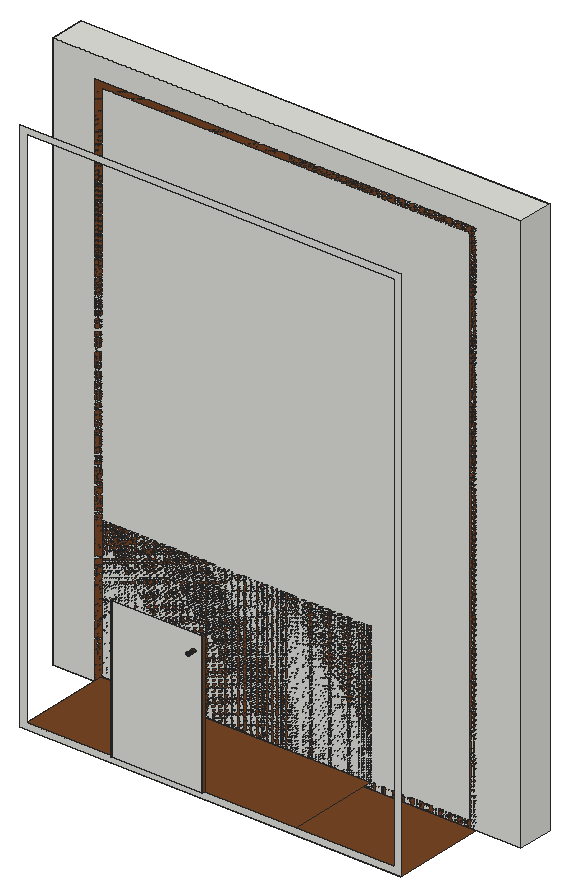
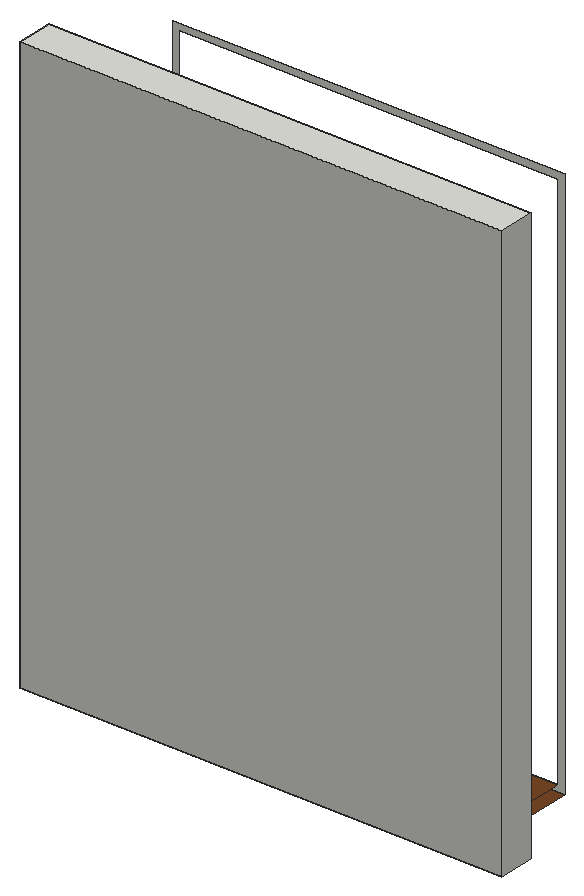
# SketchUp Ruby script. Lengths in inches.
U = 1.inch
M = Sketchup.active_model
def pt(a) = Geom::Point3d.new(a.map { |v| v * U })
def face(e, loops, mat)
  f = e.add_face(loops[0].map { |a| pt(a) })
  loops[1..].each { |l| e.add_face(l.map { |a| pt(a) }).erase! }
  f.material = f.back_material = mat if mat
  f
end
# faces: each face lists its corners as indices into pts; further lists are holes
def faces(e, pts, list, mat = nil) = list.each { |f| face(e, (f[0].is_a?(Array) ? f : [f]).map { |l| l.map { |i| pts[i] } }, mat) }
# xy, xz, yz: faces in a plane at the given z, y or x. An outline is a flat list of corners, or four numbers for a rectangle; further outlines are holes
def ring(l) = l.size == 4 ? [[l[0], l[1]], [l[2], l[1]], [l[2], l[3]], [l[0], l[3]]] : l.each_slice(2).to_a
def flat(e, list, mat, &to3) = list.each { |f| face(e, (f[0].is_a?(Array) ? f : [f]).map { |l| ring(l).map { |u, v| to3.(u, v) } }, mat) }
def xy(e, z, list, mat = nil) = flat(e, list, mat) { |x, y| [x, y, z] }
def xz(e, y, list, mat = nil) = flat(e, list, mat) { |x, z| [x, y, z] }
def yz(e, x, list, mat = nil) = flat(e, list, mat) { |y, z| [x, y, z] }
def lines(e, pts, list) = list.each { |a, b| e.add_line(pt(pts[a]), pt(pts[b])) }
# prism: a flat outline (further loops are holes) pulled along v
def prism(e, loops, v, mat = nil)
  f = face(e, loops, mat); d = Geom::Vector3d.new(v.map { |x| x * U })
  f.pushpull(f.normal.samedirection?(d) ? d.length : -d.length)
end
def box(e, o, s, mat = nil) = prism(e, [[o, [o[0] + s[0], o[1], o[2]], [o[0] + s[0], o[1] + s[1], o[2]], [o[0], o[1] + s[1], o[2]]]], [0, 0, s[2]], mat)
def at(x, y, z, deg = 0) = Geom::Transformation.translation(pt([x, y, z])) * Geom::Transformation.rotation(ORIGIN, Z_AXIS, deg.degrees)
def axes(o, x, y, z) = Geom::Transformation.new([*x, 0, *y, 0, *z, 0, *pt(o).to_a, 1])
def part(name) = M.definitions.add(name)
# library, detail: a bought-in or finely detailed component or shape, given as its bounding box
def library(name, o, s) = part(name).tap { |d| box(d.entities, o, s) }
def detail(e, o, s) = box(e.add_group.entities, o, s)
def put(e, d, t, mat = nil) = e.add_instance(d, t).tap { |i| i.material = mat if mat }
def group(e, t, mat = nil) = e.add_group.tap { |g| g.transformation = t; g.material = mat if mat }.entities
root = M.entities
M.materials.add("[Wood Veneer 01]").color = [120, 70, 37]
xy(root,0,[[10.79,2.47,108.43,26.47]],"[Wood Veneer 01]")
xy(root,1.59,[[34.5,2,57.76,2.47],[12.38,2.47,81.38,26.47]],"[Wood Veneer 01]")
xz(root,0,[[55.68,33.35,55.68,33.37,55.6,33.375,55.59,33.36],[55.68,33.35,55.77,33.36,55.76,33.375,55.68,33.37],[55.59,33.36,55.6,33.375,55.52,33.41,55.51,33.39],[55.77,33.36,55.85,33.39,55.84,33.41,55.76,33.375],[55.68,33.37,55.68,33.38,55.6,33.39,55.6,33.375],
  [55.68,33.37,55.76,33.375,55.76,33.39,55.68,33.38],[55.6,33.375,55.6,33.39,55.53,33.42,55.52,33.41],[55.76,33.375,55.84,33.41,55.83,33.42,55.76,33.39],[55.68,33.38,55.68,33.4,55.61,33.41,55.6,33.39],[55.68,33.38,55.76,33.39,55.75,33.41,55.68,33.4],
  [55.51,33.39,55.52,33.41,55.45,33.46,55.44,33.45],[55.6,33.39,55.61,33.41,55.54,33.4375,55.53,33.42],[55.76,33.39,55.83,33.42,55.82,33.4375,55.75,33.41],[55.85,33.39,55.92,33.45,55.9,33.46,55.84,33.41],[55.68,33.4,55.75,33.41,55.82,33.4375,55.88,33.48,55.92,33.54,55.95,33.61,55.96,33.68,55.95,33.76,55.92,33.82,55.88,33.88,55.82,33.93,55.75,33.96,55.68,33.97,55.61,33.96,55.54,33.93,55.48,33.88,55.43,33.82,55.41,33.76,55.4,33.68,55.41,33.61,55.43,33.54,55.48,33.48,55.54,33.4375,55.61,33.41],
  [55.52,33.41,55.53,33.42,55.47,33.47,55.45,33.46],[55.84,33.41,55.9,33.46,55.89,33.47,55.83,33.42],[55.53,33.42,55.54,33.4375,55.48,33.48,55.47,33.47],[55.83,33.42,55.89,33.47,55.88,33.48,55.82,33.4375],[55.44,33.45,55.45,33.46,55.4,33.52,55.39,33.52],
  [55.92,33.45,55.97,33.52,55.95,33.52,55.9,33.46],[55.45,33.46,55.47,33.47,55.42,33.53,55.4,33.52],[55.9,33.46,55.95,33.52,55.9375,33.53,55.89,33.47],[55.47,33.47,55.48,33.48,55.43,33.54,55.42,33.53],[55.89,33.47,55.9375,33.53,55.92,33.54,55.88,33.48],
  [55.39,33.52,55.4,33.52,55.37,33.6,55.36,33.6],[55.4,33.52,55.42,33.53,55.39,33.61,55.37,33.6],[55.95,33.52,55.99,33.6,55.97,33.61,55.9375,33.53],[55.95,33.52,55.97,33.52,56,33.6,55.99,33.6],[55.42,33.53,55.43,33.54,55.41,33.61,55.39,33.61],
  [55.9375,33.53,55.97,33.61,55.95,33.61,55.92,33.54],[55.36,33.6,55.37,33.6,55.36,33.68,55.35,33.68],[55.37,33.6,55.39,33.61,55.38,33.68,55.36,33.68],[55.99,33.6,56,33.68,55.98,33.68,55.97,33.61],[55.99,33.6,56,33.6,56.01,33.68,56,33.68],
  [55.39,33.61,55.41,33.61,55.4,33.68,55.38,33.68],[55.95,33.61,55.97,33.61,55.98,33.68,55.96,33.68],[55.38,33.68,55.4,33.68,55.41,33.76,55.39,33.76],[55.96,33.68,55.98,33.68,55.97,33.76,55.95,33.76],[55.98,33.68,56,33.68,55.99,33.77,55.97,33.76],
  [56,33.68,56.01,33.68,56,33.77,55.99,33.77]],"[Wood Veneer 01]")
xz(root,0.01,[[55.68,33.31,55.68,33.32,55.59,33.33,55.58,33.32],[55.68,33.31,55.78,33.32,55.77,33.33,55.68,33.32],[55.58,33.32,55.59,33.33,55.5,33.37,55.49,33.36],[55.68,33.32,55.68,33.33,55.59,33.35,55.59,33.33],[55.68,33.32,55.77,33.33,55.77,33.35,55.68,33.33],
  [55.78,33.32,55.87,33.36,55.86,33.37,55.77,33.33],[55.59,33.33,55.59,33.35,55.5,33.38,55.5,33.37],[55.77,33.33,55.86,33.37,55.85,33.38,55.77,33.35],[55.49,33.36,55.5,33.37,55.42,33.43,55.41,33.42],[55.87,33.36,55.95,33.42,55.9375,33.43,55.86,33.37],
  [55.5,33.37,55.5,33.38,55.43,33.4375,55.42,33.43],[55.86,33.37,55.9375,33.43,55.93,33.4375,55.85,33.38],[55.41,33.42,55.42,33.43,55.36,33.5,55.35,33.49],[55.95,33.42,56.01,33.49,55.99,33.5,55.9375,33.43],[55.42,33.43,55.43,33.4375,55.38,33.51,55.36,33.5],
  [55.9375,33.43,55.99,33.5,55.98,33.51,55.93,33.4375],[55.35,33.49,55.36,33.5,55.33,33.59,55.31,33.59],[56.01,33.49,56.04,33.59,56.03,33.59,55.99,33.5],[55.36,33.5,55.38,33.51,55.34,33.59,55.33,33.59],[55.99,33.5,56.03,33.59,56.02,33.59,55.98,33.51],
  [55.31,33.59,55.33,33.59,55.32,33.68,55.3,33.68],[55.33,33.59,55.34,33.59,55.33,33.68,55.32,33.68],[56.02,33.59,56.03,33.59,56.04,33.68,56.03,33.68],[56.03,33.59,56.04,33.59,56.06,33.68,56.04,33.68],[56.03,33.68,56.04,33.68,56.03,33.78,56.02,33.77],
  [56.04,33.68,56.06,33.68,56.04,33.78,56.03,33.78]],"[Wood Veneer 01]")
xz(root,0.02,[[55.68,33.28,55.68,33.29,55.58,33.31,55.57,33.29],[55.68,33.28,55.78,33.29,55.78,33.31,55.68,33.29],[55.57,33.29,55.58,33.31,55.48,33.34,55.48,33.33],[55.78,33.29,55.88,33.33,55.875,33.34,55.78,33.31],[55.48,33.33,55.48,33.34,55.4,33.41,55.39,33.4],
  [55.88,33.33,55.96,33.4,55.96,33.41,55.875,33.34],[55.39,33.4,55.4,33.41,55.34,33.49,55.33,33.48],[55.96,33.4,56.03,33.48,56.02,33.49,55.96,33.41],[55.33,33.48,55.34,33.49,55.3,33.58,55.29,33.58],[56.03,33.48,56.07,33.58,56.06,33.58,56.02,33.49],
  [55.29,33.58,55.3,33.58,55.29,33.68,55.28,33.68],[56.06,33.58,56.07,33.58,56.08,33.68,56.07,33.68],[56.07,33.68,56.08,33.68,56.07,33.79,56.06,33.78]],"[Wood Veneer 01]")
xz(root,0.05,[[55.68,33.24,55.68,33.25,55.57,33.26,55.5625,33.25],[55.68,33.24,55.79,33.25,55.79,33.26,55.68,33.25],[55.5625,33.25,55.57,33.26,55.46,33.31,55.46,33.3],[55.79,33.25,55.9,33.3,55.9,33.31,55.79,33.26],[55.46,33.3,55.46,33.31,55.37,33.375,55.36,33.37],
  [55.9,33.3,55.99,33.37,55.99,33.375,55.9,33.31],[55.36,33.37,55.37,33.375,55.3,33.47,55.29,33.46],[55.99,33.37,56.07,33.46,56.06,33.47,55.99,33.375],[55.29,33.46,55.3,33.47,55.26,33.57,55.25,33.57],[56.07,33.46,56.11,33.57,56.1,33.57,56.06,33.47],
  [60.23,33.5625,60.24,33.57,60.23,33.68,60.22,33.68],[55.25,33.57,55.26,33.57,55.24,33.68,55.23,33.68],[56.1,33.57,56.11,33.57,56.125,33.68,56.12,33.68],[56.12,33.68,56.125,33.68,56.11,33.8,56.1,33.8]],"[Wood Veneer 01]")
xz(root,2,[[[34.5,1.59,57.76,37.59],[55.68,33.18,55.55,33.2,55.43,33.25,55.33,33.33,55.25,33.43,55.2,33.55,55.18,33.68,55.2,33.8125,55.25,33.93,55.33,34.04,55.43,34.12,55.55,34.17,55.68,34.18,55.81,34.17,55.93,34.12,56.03,34.04,56.11,33.93,56.16,33.8125,56.18,33.68,56.16,33.55,56.11,33.43,56.03,33.33,55.93,33.25,55.81,33.2]]])
xz(root,2.47,[[[10.79,0,108.43,138.34],[12.38,1.59,106.84,136.75]]])
xz(root,2.47,[[34.26,1.59,34.5,37.59],[57.76,1.59,58,37.59]],"[Wood Veneer 01]")
xz(root,26.47,[[[10.79,0,108.43,138.34],[12.38,1.59,106.84,136.75]],[12.38,1.59,81.38,37.59]],"[Wood Veneer 01]")
yz(root,34.26,[[2,1.59,2.47,37.59]],"[Wood Veneer 01]")
yz(root,34.5,[[2,1.59,2.47,37.59]],"[Wood Veneer 01]")
yz(root,57.76,[[2,1.59,2.47,37.59]],"[Wood Veneer 01]")
yz(root,58,[[2,1.59,2.47,37.59]],"[Wood Veneer 01]")
p = [[55.57,0.05,33.26],[55.68,0.05,33.25],[55.68,0.04,33.26],[55.57,0.04,33.27],[55.79,0.04,33.27],[55.79,0.05,33.26],
  [55.55,0.15,33.21],[55.43,0.15,33.26],[55.43,0.17,33.25],[55.55,0.17,33.2],[55.55,0.14,33.21],[55.43,0.14,33.26],
  [55.55,0.12,33.21],[55.4375,0.12,33.26],[55.55,0.11,33.22],[55.4375,0.11,33.27],[55.56,0.1,33.22],[55.44,0.1,33.27],
  [55.56,0.08,33.23],[55.44,0.08,33.28],[55.56,0.07,33.24],[55.45,0.07,33.28],[55.5625,0.0625,33.24],[55.45,0.0625,33.29],
  [55.5625,0.05,33.25],[55.46,0.05,33.3],[55.68,0.17,33.1875],[55.68,0.15,33.1875],[55.68,0.14,33.19],[55.68,0.12,33.2],
  [55.68,0.11,33.2],[55.68,0.1,33.21],[55.68,0.08,33.21],[55.68,0.07,33.22],[55.68,0.0625,33.23],[55.68,0.05,33.24],
  [55.79,0.05,33.25],[55.8,0.0625,33.24],[55.8,0.07,33.24],[55.8,0.08,33.23],[55.8,0.1,33.22],[55.8,0.11,33.22],
  [55.81,0.12,33.21],[55.81,0.14,33.21],[55.81,0.15,33.21],[55.81,0.17,33.2],[55.91,0.0625,33.29],[55.9,0.05,33.3],
  [55.91,0.07,33.28],[55.91,0.08,33.28],[55.92,0.1,33.27],[55.92,0.11,33.27],[55.92,0.12,33.26],[55.92,0.14,33.26],
  [55.93,0.15,33.26],[55.93,0.17,33.25],[55.43,2,33.25],[55.55,2,33.2],[55.55,0.22,33.2],[55.43,0.22,33.25],
  [55.55,0.2,33.2],[55.43,0.2,33.25],[55.55,0.18,33.2],[55.43,0.18,33.25],[55.68,2,33.18],[55.68,0.22,33.18],
  [55.68,0.2,33.18],[55.68,0.18,33.18],[55.81,0.18,33.2],[55.81,0.2,33.2],[55.81,0.22,33.2],[55.81,2,33.2],
  [55.93,0.18,33.25],[55.93,0.2,33.25],[55.93,0.22,33.25],[55.93,2,33.25],[55.47,0.04,33.3125],[55.38,0.04,33.38],
  [55.37,0.05,33.375],[55.46,0.05,33.31],[55.47,0.03,33.32],[55.39,0.03,33.39],[55.48,0.02,33.33],[55.39,0.02,33.4],
  [55.49,0.01,33.36],[55.41,0.01,33.42],[55.4,0.02,33.41],[55.48,0.02,33.34],[55.57,0.03,33.28],[55.57,0.02,33.29],
  [55.58,0.01,33.32],[55.58,0.02,33.31],[55.59,0,33.36],[55.51,0,33.39],[55.5,0.01,33.38],[55.59,0.01,33.35],
  [55.68,0.03,33.27],[55.68,0.02,33.28],[55.68,0.02,33.29],[55.68,0.01,33.31],[55.68,0.01,33.33],[55.68,0,33.35],
  [55.77,0,33.36],[55.77,0.01,33.35],[55.78,0.01,33.32],[55.78,0.02,33.31],[55.78,0.02,33.29],[55.79,0.03,33.28],
  [55.85,0.01,33.38],[55.85,0,33.39],[55.875,0.02,33.34],[55.87,0.01,33.36],[55.89,0.03,33.32],[55.88,0.02,33.33],
  [55.89,0.04,33.3125],[55.9,0.05,33.31],[55.95,0.01,33.42],[55.96,0.02,33.41],[55.96,0.02,33.4],[55.97,0.03,33.39],
  [55.98,0.04,33.38],[55.99,0.05,33.375],[55.25,0.17,33.44],[55.33,0.17,33.33],[55.33,0.15,33.33],[55.25,0.15,33.4375],
  [55.33,0.14,33.34],[55.25,0.14,33.4375],[55.34,0.12,33.34],[55.26,0.12,33.44],[55.34,0.11,33.34],[55.26,0.11,33.44],
  [55.34,0.1,33.35],[55.27,0.1,33.45],[55.35,0.08,33.35],[55.27,0.08,33.45],[55.35,0.07,33.36],[55.36,0.0625,33.36],
  [55.36,0.05,33.37],[55.99,0.05,33.37],[56,0.0625,33.36],[56.01,0.07,33.36],[56.01,0.08,33.35],[56.02,0.1,33.35],
  [56.02,0.11,33.34],[56.02,0.12,33.34],[56.03,0.14,33.34],[56.03,0.15,33.33],[56.03,0.17,33.33],[56.09,0.1,33.45],
  [56.09,0.08,33.45],[56.1,0.11,33.44],[56.1,0.12,33.44],[56.1,0.14,33.4375],[56.11,0.15,33.4375],[56.11,0.17,33.44],
  [55.25,2,33.43],[55.33,2,33.33],[55.33,0.22,33.33],[55.25,0.22,33.43],[55.33,0.2,33.33],[55.25,0.2,33.43],
  [55.33,0.18,33.33],[55.25,0.18,33.43],[56.03,0.18,33.33],[56.03,0.2,33.33],[56.03,0.22,33.33],[56.03,2,33.33],
  [56.11,0.18,33.43],[56.11,0.2,33.43],[56.11,0.22,33.43],[56.11,2,33.43],[55.3,0.05,33.47],[55.31,0.04,33.47],
  [55.32,0.03,33.48],[55.33,0.02,33.48],[55.34,0.02,33.49],[55.35,0.01,33.49],[55.38,0.01,33.51],[55.43,0.01,33.4375],
  [55.44,0,33.45],[55.39,0,33.52],[55.92,0,33.45],[55.93,0.01,33.4375],[55.98,0.01,33.51],[55.97,0,33.52],
  [56.02,0.02,33.49],[56.01,0.01,33.49],[56.04,0.03,33.48],[56.03,0.02,33.48],[56.05,0.04,33.47],[56.06,0.05,33.47],
  [55.2,0.15,33.56],[55.2,0.17,33.55],[55.21,0.14,33.56],[55.21,0.12,33.56],[55.21,0.11,33.56],[55.22,0.1,33.56],
  [55.23,0.08,33.5625],[55.28,0.07,33.45],[55.23,0.07,33.5625],[55.29,0.0625,33.46],[55.29,0.05,33.46],[56.07,0.0625,33.46],
  [56.07,0.05,33.46],[56.08,0.07,33.45],[56.125,0.07,33.5625],[56.13,0.08,33.5625],[56.14,0.1,33.56],[56.14,0.11,33.56],
  [56.15,0.12,33.56],[56.15,0.14,33.56],[56.16,0.15,33.56],[56.16,0.17,33.55],[60.25,0.14,33.43],[60.2,0.14,33.55],
  [60.2,0.16,33.55],[60.25,0.16,33.43],[60.25,0.13,33.4375],[60.2,0.13,33.56],[60.25,0.12,33.4375],[60.2,0.12,33.56],
  [60.26,0.1,33.4375],[60.21,0.1,33.56],[60.26,0.09,33.44],[60.21,0.09,33.56],[60.26,0.08,33.44],[60.22,0.08,33.56],
  [55.2,2,33.55],[55.2,0.22,33.55],[55.2,0.2,33.55],[55.2,0.18,33.55],[56.16,0.18,33.55],[56.16,0.2,33.55],
  [56.16,0.22,33.55],[56.16,2,33.55],[60.2,2,33.55],[60.25,2,33.43],[60.25,0.19,33.43],[60.2,0.19,33.55],
  [60.25,0.17,33.43],[60.2,0.17,33.55],[55.27,0.04,33.57],[55.26,0.05,33.57],[55.28,0.03,33.58],[55.29,0.02,33.58],
  [55.31,0.01,33.59],[55.3,0.02,33.58],[55.36,0,33.6],[55.34,0.01,33.59],[56,0,33.6],[56.02,0.01,33.59],
  [56.04,0.01,33.59],[56.06,0.02,33.58],[56.07,0.02,33.58],[56.08,0.03,33.58],[56.09,0.04,33.57],[56.1,0.05,33.57],
  [55.24,0.0625,33.57],[55.25,0.05,33.57],[56.11,0.05,33.57],[56.12,0.0625,33.57],[55.24,0.05,33.68],[55.25,0.04,33.68],
  [55.26,0.03,33.68],[55.28,0.02,33.68],[55.29,0.02,33.68],[55.3,0.01,33.68],[55.33,0.01,33.68],[55.35,0,33.68],
  [56.03,0.01,33.68],[56.01,0,33.68],[56.07,0.02,33.68],[56.06,0.01,33.68],[56.09,0.03,33.68],[56.08,0.02,33.68],
  [56.11,0.04,33.68],[56.12,0.05,33.68],[60.25,0.04,33.57],[60.23,0.04,33.68],[60.23,0.05,33.68],[60.24,0.05,33.57],
  [55.18,0.17,33.68],[55.19,0.15,33.68],[55.1875,0.14,33.68],[55.19,0.12,33.68],[55.2,0.11,33.68],[55.2,0.1,33.68],
  [55.21,0.08,33.68],[55.22,0.07,33.68],[55.23,0.0625,33.68],[55.23,0.05,33.68],[56.13,0.0625,33.68],[56.125,0.05,33.68],
  [56.14,0.07,33.68],[56.15,0.08,33.68],[56.16,0.1,33.68],[56.16,0.11,33.68],[56.17,0.12,33.68],[56.17,0.14,33.68],
  [56.17,0.15,33.68],[56.18,0.17,33.68],[60.18,0.14,33.68],[60.18,0.16,33.68],[60.18,0.13,33.68],[60.1875,0.12,33.68],
  [60.19,0.1,33.68],[60.2,0.09,33.68],[60.2,0.08,33.68],[60.22,0.07,33.5625],[60.21,0.07,33.68],[60.23,0.0625,33.5625],
  [60.21,0.0625,33.68],[60.23,0.05,33.5625],[60.22,0.05,33.68],[33.16,2,33.55],[33.18,2,33.68],[33.18,0.21,33.68],
  [33.16,0.21,33.55],[55.18,2,33.68],[55.18,0.22,33.68],[55.18,0.2,33.68],[55.18,0.18,33.68],[56.18,0.18,33.68],
  [56.18,0.2,33.68],[56.18,0.22,33.68],[56.18,2,33.68],[60.18,2,33.68],[60.18,0.19,33.68],[60.18,0.17,33.68],
  [56,0,33.77],[56.02,0.01,33.77],[56.04,0.01,33.78],[56.06,0.02,33.78],[56.07,0.02,33.79],[56.08,0.03,33.79],
  [56.09,0.04,33.79],[56.1,0.05,33.8],[33.16,2,33.8125],[33.16,0.21,33.8125],[55.2,0.18,33.8125],[55.2,0.2,33.8125],
  [55.2,0.17,33.8125]]
faces(root,p,[[0,1,2,3],[4,2,1,5],[6,7,8,9],[10,11,7,6],[12,13,11,10],[14,15,13,12],[16,17,15,14],[18,19,17,16],
  [20,21,19,18],[22,23,21,20],[24,25,23,22],[9,26,27,6],[6,27,28,10],[10,28,29,12],[12,29,30,14],[14,30,31,16],
  [16,31,32,18],[18,32,33,20],[20,33,34,22],[22,34,35,24],[36,35,34,37],[37,34,33,38],[38,33,32,39],[39,32,31,40],
  [40,31,30,41],[41,30,29,42],[42,29,28,43],[43,28,27,44],[44,27,26,45],[37,46,47,36],[38,48,46,37],[39,49,48,38],
  [40,50,49,39],[41,51,50,40],[42,52,51,41],[43,53,52,42],[44,54,53,43],[45,55,54,44],[56,57,58,59],[60,61,59,58],
  [62,63,61,60],[9,8,63,62],[57,64,65,58],[58,65,66,60],[60,66,67,62],[62,67,26,9],[45,26,67,68],[68,67,66,69],
  [69,66,65,70],[64,71,70,65],[68,72,55,45],[69,73,72,68],[70,74,73,69],[71,75,74,70],[76,77,78,79],[80,81,77,76],
  [82,83,81,80],[84,85,86,87],[3,76,79,0],[88,80,76,3],[89,82,80,88],[90,84,87,91],[92,93,94,95],[3,2,96,88],
  [88,96,97,89],[91,98,99,90],[95,100,101,92],[102,101,100,103],[104,99,98,105],[106,97,96,107],[107,96,2,4],[103,108,109,102],
  [105,110,111,104],[107,112,113,106],[4,114,112,107],[5,115,114,4],[116,111,110,117],[118,113,112,119],[119,112,114,120],[120,114,115,121],
  [122,123,124,125],[125,124,126,127],[127,126,128,129],[129,128,130,131],[131,130,132,133],[133,132,134,135],[7,124,123,8],[11,126,124,7],
  [13,128,126,11],[15,130,128,13],[17,132,130,15],[19,134,132,17],[21,136,134,19],[23,137,136,21],[25,138,137,23],[139,47,46,140],
  [140,46,48,141],[141,48,49,142],[142,49,50,143],[143,50,51,144],[144,51,52,145],[145,52,53,146],[146,53,54,147],[147,54,55,148],
  [143,149,150,142],[144,151,149,143],[145,152,151,144],[146,153,152,145],[147,154,153,146],[148,155,154,147],[156,157,158,159],[159,158,160,161],
  [161,160,162,163],[163,162,123,122],[157,56,59,158],[61,160,158,59],[63,162,160,61],[8,123,162,63],[148,55,72,164],[164,72,73,165],
  [165,73,74,166],[75,167,166,74],[164,168,155,148],[165,169,168,164],[166,170,169,165],[167,171,170,166],[172,78,77,173],[173,77,81,174],
  [174,81,83,175],[176,86,85,177],[178,179,180,181],[93,180,179,94],[182,109,108,183],[183,184,185,182],[117,186,187,116],[119,188,189,118],
  [120,190,188,119],[121,191,190,120],[125,192,193,122],[127,194,192,125],[129,195,194,127],[131,196,195,129],[133,197,196,131],[135,198,197,133],
  [199,200,198,135],[135,134,136,199],[199,136,137,201],[201,137,138,202],[140,203,204,139],[141,205,203,140],[142,150,205,141],[206,205,150,207],
  [207,150,149,208],[208,149,151,209],[209,151,152,210],[210,152,153,211],[211,153,154,212],[212,154,155,213],[214,215,216,217],[218,219,215,214],
  [220,221,219,218],[222,223,221,220],[224,225,223,222],[226,227,225,224],[228,156,159,229],[161,230,229,159],[163,231,230,161],[122,193,231,163],
  [213,155,168,232],[232,168,169,233],[233,169,170,234],[171,235,234,170],[236,237,238,239],[240,241,239,238],[217,216,241,240],[173,242,243,172],
  [174,244,242,173],[175,245,244,174],[177,246,247,176],[181,248,249,178],[250,185,184,251],[252,187,186,253],[254,189,188,255],[255,188,190,256],
  [256,190,191,257],[201,258,200,199],[202,259,258,201],[260,204,203,261],[261,203,205,206],[262,243,242,263],[263,242,244,264],[264,244,245,265],
  [266,247,246,267],[268,249,248,269],[251,270,271,250],[253,272,273,252],[255,274,275,254],[256,276,274,255],[257,277,276,256],[278,279,280,281],
  [282,193,192,283],[283,192,194,284],[284,194,195,285],[285,195,196,286],[286,196,197,287],[287,197,198,288],[288,198,200,289],[289,200,258,290],
  [290,258,259,291],[261,292,293,260],[206,294,292,261],[207,295,294,206],[208,296,295,207],[209,297,296,208],[210,298,297,209],[211,299,298,210],
  [212,300,299,211],[213,301,300,212],[215,302,303,216],[219,304,302,215],[221,305,304,219],[223,306,305,221],[225,307,306,223],[227,308,307,225],
  [309,310,308,227],[311,312,310,309],[313,314,312,311],[315,316,317,318],[319,228,229,320],[320,229,230,321],[321,230,231,322],[322,231,193,282],
  [232,323,301,213],[233,324,323,232],[234,325,324,233],[235,326,325,234],[327,236,239,328],[241,329,328,239],[216,303,329,241],[330,271,270,331],
  [332,273,272,333],[334,275,274,335],[335,274,276,336],[336,276,277,337],[316,338,339,317],[322,340,341,321],[282,342,340,322]],"[Wood Veneer 01]")
g1 = group(root,at(0,26.47,0))
box(g1,[0,0,0],[120,9,144])
